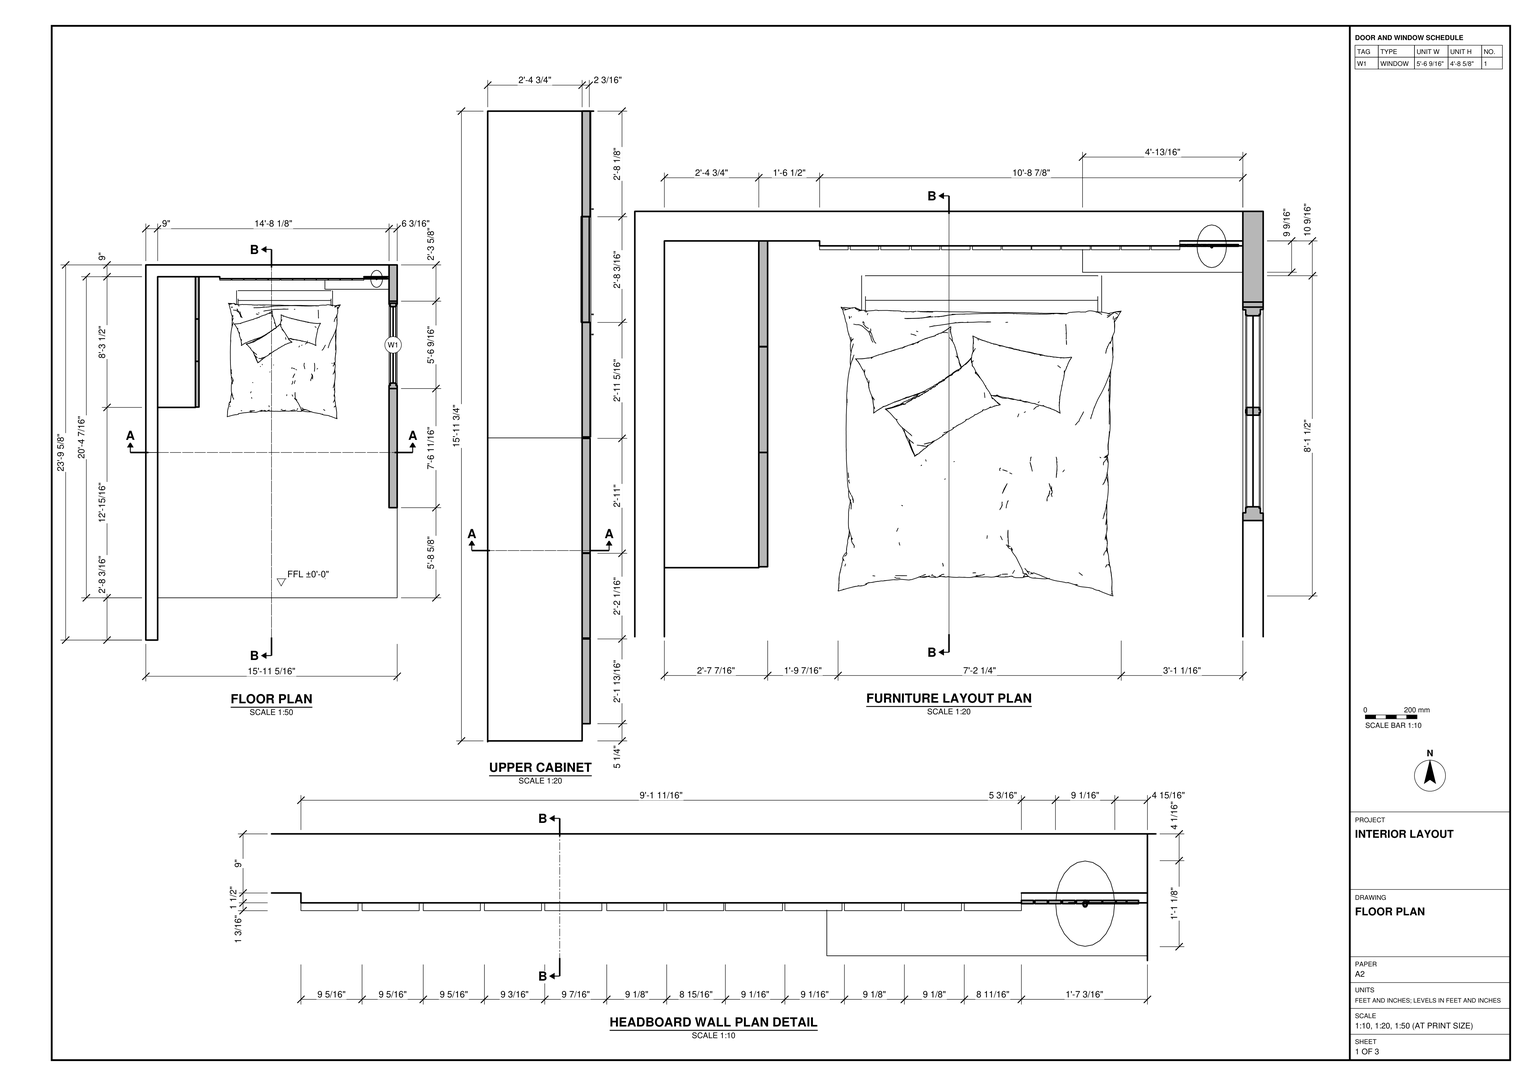
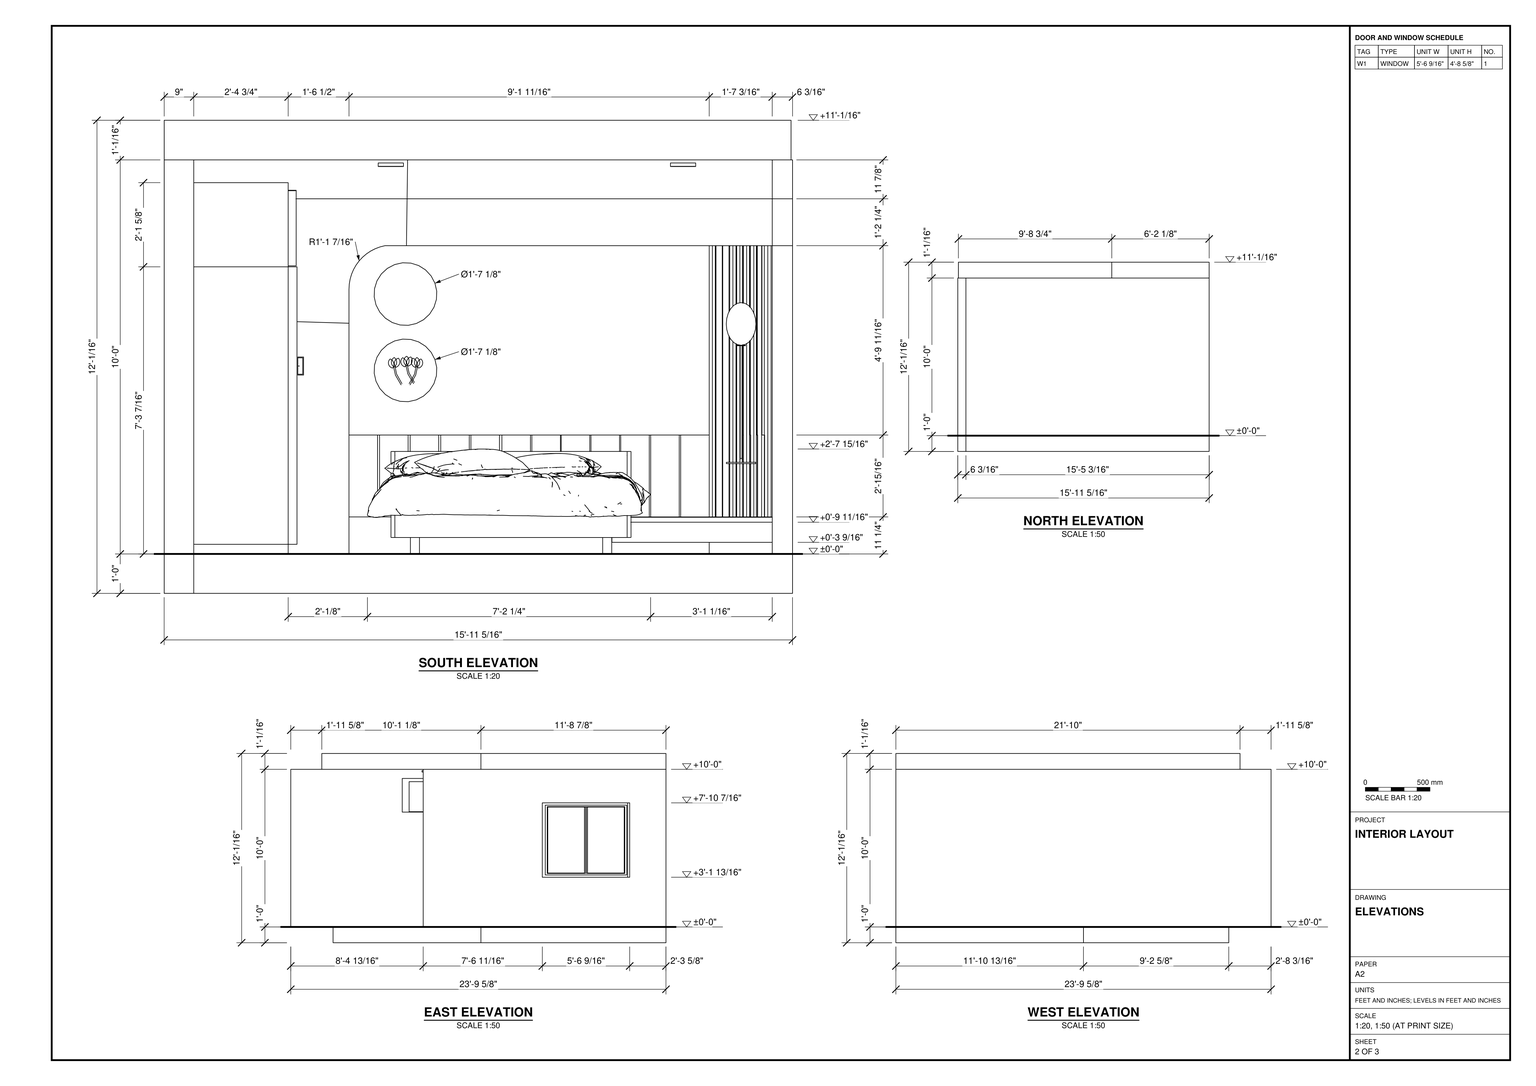
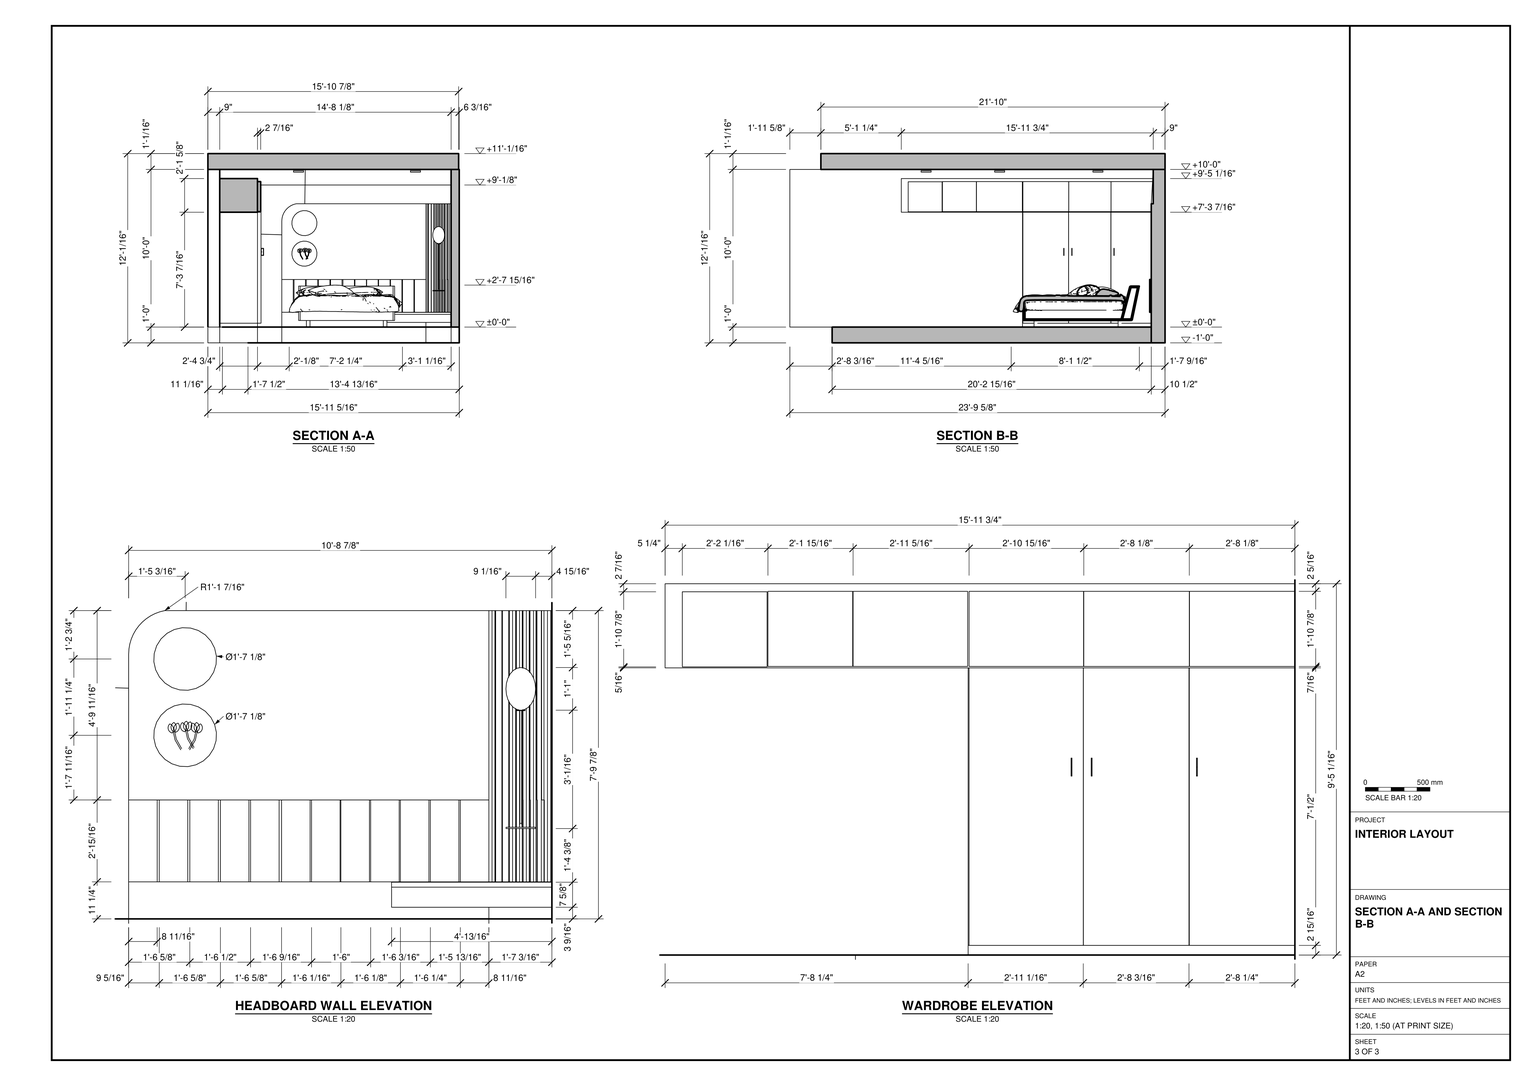
Build the bedroom interior in SketchUp using task_files/diagram_01.pdf. Work in feet and inches. The overall model is 15'-11 5/16" wide, 23'-9 5/8" long and 12'-1/16" high, with the finished floor at ±0'-0". Follow the floor plan for the wall thicknesses and unequal side-wall lengths. Leave the south end open as drawn. Use the sections to set out the floor slab and flat roof slab, noting that their ends do not align. Fit the framed window assembly into the east wall beside the bed.

Place the platform bed with its head toward the north wall, leaving the clearances shown between the bed, wardrobe and window wall. Along the west wall, model the tall wardrobe doors and handles beneath the row of upper cupboards. Continue the upper cupboards beyond the tall doors toward the open end. Behind the bed, model the broad panel with its rounded upper left corner, the divided panels below it, the narrow slatted section on the right and the low projecting shelf. Decor and loose items may be any suitable library components placed as shown.

Keep each shell element and each furniture or joinery piece in a separate group or component, and use components for repeated parts. Save one SketchUp model as output_files/bedroom_with_a_fitted_wardrobe_and_headboard_wall.skp.

# SketchUp Ruby script. Lengths in inches.
U = 1.inch
M = Sketchup.active_model
def pt(a) = Geom::Point3d.new(a.map { |v| v * U })
def face(e, loops, mat)
  f = e.add_face(loops[0].map { |a| pt(a) })
  loops[1..].each { |l| e.add_face(l.map { |a| pt(a) }).erase! }
  f.material = f.back_material = mat if mat
  f
end
# faces: each face lists its corners as indices into pts; further lists are holes
def faces(e, pts, list, mat = nil) = list.each { |f| face(e, (f[0].is_a?(Array) ? f : [f]).map { |l| l.map { |i| pts[i] } }, mat) }
# xy, xz, yz: faces in a plane at the given z, y or x. An outline is a flat list of corners, or four numbers for a rectangle; further outlines are holes
def ring(l) = l.size == 4 ? [[l[0], l[1]], [l[2], l[1]], [l[2], l[3]], [l[0], l[3]]] : l.each_slice(2).to_a
def flat(e, list, mat, &to3) = list.each { |f| face(e, (f[0].is_a?(Array) ? f : [f]).map { |l| ring(l).map { |u, v| to3.(u, v) } }, mat) }
def xy(e, z, list, mat = nil) = flat(e, list, mat) { |x, y| [x, y, z] }
def xz(e, y, list, mat = nil) = flat(e, list, mat) { |x, z| [x, y, z] }
def yz(e, x, list, mat = nil) = flat(e, list, mat) { |y, z| [x, y, z] }
def lines(e, pts, list) = list.each { |a, b| e.add_line(pt(pts[a]), pt(pts[b])) }
# prism: a flat outline (further loops are holes) pulled along v
def prism(e, loops, v, mat = nil)
  f = face(e, loops, mat); d = Geom::Vector3d.new(v.map { |x| x * U })
  f.pushpull(f.normal.samedirection?(d) ? d.length : -d.length)
end
def box(e, o, s, mat = nil) = prism(e, [[o, [o[0] + s[0], o[1], o[2]], [o[0] + s[0], o[1] + s[1], o[2]], [o[0], o[1] + s[1], o[2]]]], [0, 0, s[2]], mat)
def at(x, y, z, deg = 0) = Geom::Transformation.translation(pt([x, y, z])) * Geom::Transformation.rotation(ORIGIN, Z_AXIS, deg.degrees)
def axes(o, x, y, z) = Geom::Transformation.new([*x, 0, *y, 0, *z, 0, *pt(o).to_a, 1])
def part(name) = M.definitions.add(name)
# library, detail: a bought-in or finely detailed component or shape, given as its bounding box
def library(name, o, s) = part(name).tap { |d| box(d.entities, o, s) }
def detail(e, o, s) = box(e.add_group.entities, o, s)
def put(e, d, t, mat = nil) = e.add_instance(d, t).tap { |i| i.material = mat if mat }
def group(e, t, mat = nil) = e.add_group.tap { |g| g.transformation = t; g.material = mat if mat }.entities
root = M.entities
M.materials.add("[Carrera Marble]").color = [207, 207, 207]
M.materials.add("[Color A02]").color = [255, 153, 153]
M.materials.add("[Color M03]").color = [170, 170, 170]
M.materials.add("[CoolGray8]").color = [76, 80, 93]
M.materials.add("[Translucent Glass Gray]").color = [128, 128, 128]
M.materials["[Translucent Glass Gray]"].alpha = 0.5
M.materials.add("[Wood Cherry Original]").color = [152, 86, 42]
M.materials.add("[Wood Floor]").color = [155, 105, 61]
c1 = library("BED+04",[-44.14,-47.125,0],[86.23,97.52,31.95])
c2 = part("window full")
xy(c2.entities,0,[[0,0,14.17,66.54]])
xy(c2.entities,2.26,[[12.2,2.26,14.17,64.28]],"[Wood Floor]")
xy(c2.entities,2.36,[[0,2.36,1.97,64.17]],"[Wood Floor]")
xy(c2.entities,3.74,[[11.42,3.74,12.2,32.875],[11.42,33.66,12.2,62.79]],"[Wood Floor]")
xy(c2.entities,3.9375,[[1.97,3.9375,2.76,32.77],[1.97,33.76,2.76,62.6]],"[Wood Floor]")
xy(c2.entities,4.18,[[2.76,4.18,7.09,32.09],[7.09,4.18,11.42,32.09],[2.76,34.45,7.09,62.35],[7.09,34.45,11.42,62.35]],"[Wood Floor]")
xy(c2.entities,69.83,[[2.76,4.18,7.09,32.09],[7.09,32.09,11.42,34.45],[2.76,34.45,7.09,62.35]])
xy(c2.entities,69.83,[[7.09,4.18,11.42,32.09],[7.09,34.45,11.42,62.35]],"[Wood Floor]")
xy(c2.entities,70.08,[[1.97,3.9375,2.76,32.77],[1.97,33.76,2.76,62.6]])
xy(c2.entities,70.27,[[11.42,32.875,12.2,33.66]])
xy(c2.entities,70.27,[[11.42,3.74,12.2,32.875],[11.42,33.66,12.2,62.79]],"[Wood Floor]")
xy(c2.entities,71.65,[[0,2.36,1.97,64.17]])
xy(c2.entities,71.76,[[12.2,2.26,14.17,64.28]],"[Wood Floor]")
xy(c2.entities,74.02,[[0,0,14.17,66.54]],"[Wood Floor]")
xz(c2.entities,0,[[0,0,14.17,74.02]],"[Wood Floor]")
xz(c2.entities,2.26,[[12.2,2.26,14.17,71.76]],"[Wood Floor]")
xz(c2.entities,2.36,[[0,2.36,1.97,71.65]],"[Wood Floor]")
xz(c2.entities,3.74,[[11.42,3.74,12.2,70.27]],"[Wood Floor]")
xz(c2.entities,3.9375,[[1.97,3.9375,2.76,70.08]],"[Wood Floor]")
xz(c2.entities,4.18,[[2.76,4.18,7.09,69.83],[7.09,4.18,11.42,69.83]],"[Wood Floor]")
xz(c2.entities,32.09,[[2.76,4.18,11.42,69.83]],"[Wood Floor]")
xz(c2.entities,32.77,[[1.97,3.9375,2.76,70.08]],"[Wood Floor]")
xz(c2.entities,32.875,[[11.42,3.74,12.2,70.27]],"[Wood Floor]")
xz(c2.entities,33.66,[[11.42,3.74,12.2,47.88],[11.42,47.88,12.2,70.27]],"[Wood Floor]")
xz(c2.entities,33.76,[[1.97,3.9375,2.76,70.08]],"[Wood Floor]")
xz(c2.entities,34.45,[[2.76,4.18,11.42,69.83]],"[Wood Floor]")
xz(c2.entities,62.35,[[2.76,4.18,7.09,69.83],[7.09,4.18,11.42,69.83]],"[Wood Floor]")
xz(c2.entities,62.6,[[1.97,3.9375,2.76,70.08]],"[Wood Floor]")
xz(c2.entities,62.79,[[11.42,3.74,12.2,70.27]],"[Wood Floor]")
xz(c2.entities,64.17,[[0,2.36,1.97,71.65]],"[Wood Floor]")
xz(c2.entities,64.28,[[12.2,2.26,14.17,71.76]],"[Wood Floor]")
xz(c2.entities,66.54,[[0,0,14.17,74.02]],"[Wood Floor]")
yz(c2.entities,0,[[[0,0,66.54,74.02],[2.36,2.36,64.17,71.65]]],"[Wood Floor]")
yz(c2.entities,1.97,[[[2.36,2.36,64.17,71.65],[33.76,3.9375,62.6,70.08],[3.9375,3.9375,32.77,70.08]]],"[Wood Floor]")
yz(c2.entities,2.76,[[32.77,3.9375,33.76,4.18],[32.77,4.18,33.76,69.83],[32.77,69.83,33.76,70.08]])
yz(c2.entities,2.76,[[[3.9375,3.9375,32.77,70.08],[4.18,4.18,32.09,69.83]],[[33.76,3.9375,62.6,70.08],[34.45,4.18,62.35,69.83]]],"[Wood Floor]")
yz(c2.entities,7.09,[[4.18,4.18,62.35,69.83]],"[Translucent Glass Gray]")
yz(c2.entities,11.42,[[32.875,69.83,33.66,70.27]])
yz(c2.entities,11.42,[[[3.74,3.74,32.875,70.27],[4.18,4.18,32.09,69.83]],[[33.66,3.74,62.79,70.27],[34.45,4.18,62.35,69.83]]],"[Wood Floor]")
yz(c2.entities,12.2,[[[2.26,2.26,64.28,71.76],[3.74,3.74,32.875,70.27],[33.66,3.74,62.79,70.27]]],"[Wood Floor]")
yz(c2.entities,14.17,[[[0,0,66.54,74.02],[2.26,2.26,64.28,71.76]]],"[Wood Floor]")
p = [[11.42,32.875,70.27],[11.42,32.875,70.28]]
lines(c2.entities,p,[[0,1]])
c3 = library("stand lighting1",[-0.05,-6.55,3.35],[13.1,13.1,49.02])
c4 = part("Handle")
prism(c4.entities,[[[0,0,5.25],[0,0,5.5],[0,1.75,5.5],[0,1.75,0],[0,0,0],[0,0,0.25],[0,1.5,0.25],[0,1.5,5.25]]],[0.25,0,0],"[CoolGray8]")
p = [[0.25,0,0.25],[0.25,0,2.75],[0,0,0.25],[0,0,2.75],[0.25,0,5.25],[0,0,5.25],
  [0.125,0,2.75],[0.125,0.5,2.75]]
lines(c4.entities,p,[[0,1],[2,3],[1,4],[3,5],[1,6],[6,3],[6,7]])
c5 = part("グループ\#88")
xy(c5.entities,0,[[5.91,0,4.38,0.2,2.95,0.79,1.73,1.73,0.79,2.95,0.2,4.38,0,5.91,0.2,7.43,0.79,8.86,1.73,10.08,2.95,11.02,4.38,11.61,5.91,11.8125,7.43,11.61,8.86,11.02,10.08,10.08,11.02,8.86,11.61,7.43,11.8125,5.91,11.61,4.38,11.02,2.95,10.08,1.73,8.86,0.79,7.43,0.2]])
xy(c5.entities,1.57,[[5.91,0.41,7.33,0.6,8.65,1.15,9.79,2.02,10.67,3.16,11.21,4.48,11.4,5.91,11.21,7.33,10.67,8.65,9.79,9.79,8.65,10.67,7.33,11.21,5.91,11.4,4.48,11.21,3.16,10.67,2.02,9.79,1.15,8.65,0.6,7.33,0.41,5.91,0.6,4.48,1.15,3.16,2.02,2.02,3.16,1.15,4.48,0.6]])
xy(c5.entities,1.69,[[[5.91,0,7.43,0.2,8.86,0.79,10.08,1.73,11.02,2.95,11.61,4.38,11.8125,5.91,11.61,7.43,11.02,8.86,10.08,10.08,8.86,11.02,7.43,11.61,5.91,11.8125,4.38,11.61,2.95,11.02,1.73,10.08,0.79,8.86,0.2,7.43,0,5.91,0.2,4.38,0.79,2.95,1.73,1.73,2.95,0.79,4.38,0.2],[5.91,0.41,4.48,0.6,3.16,1.15,2.02,2.02,1.15,3.16,0.6,4.48,0.41,5.91,0.6,7.33,1.15,8.65,2.02,9.79,3.16,10.67,4.48,11.21,5.91,11.4,7.33,11.21,8.65,10.67,9.79,9.79,10.67,8.65,11.21,7.33,11.4,5.91,11.21,4.48,10.67,3.16,9.79,2.02,8.65,1.15,7.33,0.6]]])
p = [[4.38,0.2,0],[5.91,0,0],[5.91,0,1.69],[4.38,0.2,1.69],[7.43,0.2,0],[7.43,0.2,1.69],
  [2.95,0.79,0],[2.95,0.79,1.69],[8.86,0.79,0],[8.86,0.79,1.69],[1.73,1.73,0],[1.73,1.73,1.69],
  [10.08,1.73,0],[10.08,1.73,1.69],[0.79,2.95,0],[0.79,2.95,1.69],[11.02,2.95,0],[11.02,2.95,1.69],
  [0.2,4.38,0],[0.2,4.38,1.69],[11.61,4.38,0],[11.61,4.38,1.69],[0,5.91,0],[0,5.91,1.69],
  [11.8125,5.91,0],[11.8125,5.91,1.69],[0.2,7.43,0],[0.2,7.43,1.69],[11.61,7.43,0],[11.61,7.43,1.69],
  [0.79,8.86,0],[0.79,8.86,1.69],[11.02,8.86,0],[11.02,8.86,1.69],[1.73,10.08,0],[1.73,10.08,1.69],
  [10.08,10.08,0],[10.08,10.08,1.69],[2.95,11.02,0],[2.95,11.02,1.69],[8.86,11.02,0],[8.86,11.02,1.69],
  [4.38,11.61,0],[4.38,11.61,1.69],[7.43,11.61,0],[7.43,11.61,1.69],[5.91,11.8125,0],[5.91,11.8125,1.69],
  [4.48,0.6,1.69],[5.91,0.41,1.69],[5.91,0.41,1.57],[4.48,0.6,1.57],[7.33,0.6,1.69],[7.33,0.6,1.57],
  [3.16,1.15,1.69],[3.16,1.15,1.57],[8.65,1.15,1.69],[8.65,1.15,1.57],[2.02,2.02,1.69],[2.02,2.02,1.57],
  [9.79,2.02,1.69],[9.79,2.02,1.57],[1.15,3.16,1.69],[1.15,3.16,1.57],[10.67,3.16,1.69],[10.67,3.16,1.57],
  [0.6,4.48,1.69],[0.6,4.48,1.57],[11.21,4.48,1.69],[11.21,4.48,1.57],[0.41,5.91,1.69],[0.41,5.91,1.57],
  [11.4,5.91,1.69],[11.4,5.91,1.57],[0.6,7.33,1.69],[0.6,7.33,1.57],[11.21,7.33,1.69],[11.21,7.33,1.57],
  [1.15,8.65,1.69],[1.15,8.65,1.57],[10.67,8.65,1.69],[10.67,8.65,1.57],[2.02,9.79,1.69],[2.02,9.79,1.57],
  [9.79,9.79,1.69],[9.79,9.79,1.57],[3.16,10.67,1.69],[3.16,10.67,1.57],[8.65,10.67,1.69],[8.65,10.67,1.57],
  [4.48,11.21,1.69],[4.48,11.21,1.57],[7.33,11.21,1.69],[7.33,11.21,1.57],[5.91,11.4,1.69],[5.91,11.4,1.57]]
faces(c5.entities,p,[[0,1,2,3],[1,4,5,2],[6,0,3,7],[4,8,9,5],[10,6,7,11],[8,12,13,9],[14,10,11,15],[12,16,17,13],
  [18,14,15,19],[16,20,21,17],[22,18,19,23],[20,24,25,21],[26,22,23,27],[24,28,29,25],[30,26,27,31],[28,32,33,29],
  [34,30,31,35],[32,36,37,33],[38,34,35,39],[36,40,41,37],[42,38,39,43],[40,44,45,41],[46,42,43,47],[44,46,47,45],
  [48,49,50,51],[49,52,53,50],[54,48,51,55],[52,56,57,53],[58,54,55,59],[56,60,61,57],[62,58,59,63],[60,64,65,61],
  [66,62,63,67],[64,68,69,65],[70,66,67,71],[68,72,73,69],[74,70,71,75],[72,76,77,73],[78,74,75,79],[76,80,81,77],
  [82,78,79,83],[80,84,85,81],[86,82,83,87],[84,88,89,85],[90,86,87,91],[88,92,93,89],[94,90,91,95],[92,94,95,93]])
c6 = part("CL OL251733")
put(c6.entities,c5,axes([4.91,11.8125,72.56],[1,0,0],[0,-1,0],[0,0,-1]))
c7 = part("Group\#2")
box(c7.entities,[0,-1.1875,0],[8.69,1.1875,24.94])
c8 = part("Group\#17")
prism(c8.entities,[[[0,32.15,67.88],[0,32.15,0],[0,0,0],[0,0,84.5],[0,32.15,84.5]]],[2.6875,0,0])
c9 = part("Group\#21")
box(c9.entities,[0,0,0],[2.4375,34.875,22.875])
c10 = part("Group\#16")
box(c10.entities,[0,0,0],[2.4375,32.1875,22.875])
c11 = part("Group\#20")
box(c11.entities,[0,9.06,0],[2.4375,25.82,22.875])
c12 = part("Group\#22")
xy(c12.entities,0,[[0.875,0,1.09,0.18,1.27,0.39,1.42,0.63,1.53,0.89,1.6,1.16,1.62,1.4375,1.6,1.72,1.53,1.99,1.42,2.25,1.27,2.48,1.09,2.7,0.875,2.875,0.625,2.72,0.41,2.52,0.24,2.28,0.11,2.01,0.03,1.73,0,1.4375,0.03,1.14,0.11,0.86,0.24,0.6,0.41,0.36,0.625,0.16]])
xy(root,-12,[[9,32.1875,9,276.625,56.27,276.625,56.27,275.125,185.15,275.125,185.15,144.75,191.34,144.75,191.34,32.1875],[0,142.8125,0,285.625,185.15,285.625,185.15,276.625,165.96,276.625,165.96,275.125,56.27,275.125,56.27,276.625,9,276.625,9,142.8125],[185.15,144.75,191.34,285.625]])
xy(root,0,[[0,0,9,142.8125],[9,32.1875,191.34,32.1875,191.34,100.8125,185.15,100.8125,185.15,275.125,56.27,275.125,56.27,276.625,9,276.625],[185.15,100.8125,191.34,144.75],[165.96,275.125,185.15,276.625]])
xy(root,3.54,[[136.34,267.0625,165.96,275.125],[165.96,267.0625,185.15,275.125]])
xy(root,9.66,[[136.34,267.0625,185.15,275.125]])
xy(root,11.16,[[136.34,267.0625,185.15,275.125]],"[Wood Cherry Original]")
xy(root,37.84,[[185.15,191.47,191.34,256.47]])
xy(root,93.875,[[67.22,275.125,165.96,276.625],[165.96,275.125,185.15,276.625]])
xy(root,94.47,[[185.15,191.47,191.34,256.47]])
xy(root,120,[[0,0,9,23.625],[0,23.625,9,276.625],[9,23.625,9,276.625,185.15,276.625,185.15,100.8125,190.875,100.8125,190.875,23.625],[185.15,100.8125,190.875,285.625],[190.875,100.8125,191.34,285.625],
  [0,276.625,74.125,285.625],[74.125,276.625,185.15,285.625]])
xy(root,132.0625,[[0,23.625,190.875,285.625]])
xz(root,0,[[0,0,9,120]])
xz(root,23.625,[[0,120,190.875,132.0625]])
xz(root,32.1875,[[9,-12,191.34,0]])
xz(root,100.8125,[[185.15,0,191.34,93.875],[185.15,93.875,191.34,108.15],[185.15,108.15,191.34,120]])
xz(root,142.8125,[[0,-12,9,0]])
xz(root,144.75,[[185.15,-12,191.34,0]])
xz(root,191.47,[[185.15,37.84,191.34,94.47]])
xz(root,256.47,[[185.15,37.84,191.34,94.47]])
xz(root,267.0625,[[136.34,3.54,185.15,9.66]])
xz(root,267.0625,[[136.34,9.66,185.15,11.16]],"[Wood Cherry Original]")
xz(root,275.125,[[56.27,-12,165.96,0],[165.96,-12,185.15,0],[136.34,9.66,185.15,11.16],[64.96,11.27,165.96,36.22],[74.32,69.625,76.76,70.17,78.97,71.33,80.81,73.02,82.14,75.13,82.89,77.51,82.99,80.01,82.44,82.44,81.28,84.65,79.59,86.49,77.48,87.83,75.1,88.57,72.61,88.67,70.17,88.125,67.96,86.97,66.12,85.28,64.79,83.17,64.04,80.78,63.94,78.29,64.49,75.85,65.65,73.64,67.34,71.81,69.45,70.47,71.83,69.73]])
xz(root,275.125,[[[56.27,36.22,165.96,36.22,165.96,93.875,67.22,93.875,65.72,93.5,64.27,92.96,62.89,92.25,61.6,91.39,60.42,90.38,59.36,89.25,58.44,88,57.68,86.65,57.07,85.23,56.625,83.74,56.36,82.22,56.27,80.67],[74.32,69.625,71.83,69.73,69.45,70.47,67.34,71.81,65.65,73.64,64.49,75.85,63.94,78.29,64.04,80.78,64.79,83.17,66.12,85.28,67.96,86.97,70.17,88.125,72.61,88.67,75.1,88.57,77.48,87.83,79.59,86.49,81.28,84.65,82.44,82.44,82.99,80.01,82.89,77.51,82.14,75.13,80.81,73.02,78.97,71.33,76.76,70.17],[75.49,52.59,75.24,53.03,75.49,53.47,75.74,53.02]],[75.49,52.59,75.74,53.02,75.49,53.47,75.24,53.03]],"[Color A02]")
xz(root,275.125,[[56.27,0,165.96,0,165.96,3.54,136.34,3.54,136.34,11.16,185.15,11.16,185.15,11.27,56.27,11.27],[165.96,0,185.15,3.54],[173.17,11.27,174.23,93.875],[175.3,11.27,176.36,93.875],[176.36,11.27,177.36,93.875],
  [177.36,11.27,178.48,93.875],[178.48,11.27,179.55,93.875],[179.55,11.27,180.61,93.875],[180.61,11.27,182.73,93.875],[182.73,11.27,183.8,93.875],
  [183.8,11.27,184.8,93.875],[184.8,11.27,185.15,93.875]],"[Wood Cherry Original]")
xz(root,276.625,[[9,-12,37.75,0],[37.75,-12,56.27,0],[165.96,-12,185.15,0]])
xz(root,276.625,[[9,0,56.27,0,56.27,80.67,56.36,82.22,56.625,83.74,57.07,85.23,57.68,86.65,58.44,88,59.36,89.25,60.42,90.38,61.6,91.39,62.89,92.25,64.27,92.96,65.72,93.5,67.22,93.875,185.15,93.875,185.15,108.15,9,108.15],[9,108.15,185.15,120]],"[Carrera Marble]")
xz(root,276.625,[[165.96,0,185.15,93.875]],"[Wood Cherry Original]")
xz(root,285.625,[[0,-12,185.15,120],[185.15,-12,191.34,120],[0,120,74.125,132.0625],[74.125,120,190.875,132.0625]])
yz(root,0,[[142.8125,-12,142.8125,0,0,0,0,120,285.625,120,285.625,-12],[23.625,120,285.625,132.0625]])
yz(root,9,[[32.1875,-12,142.8125,0],[142.8125,-12,276.625,0],[0,0,276.625,120]])
yz(root,56.27,[[275.125,-12,276.625,0],[275.125,0,276.625,80.67]])
yz(root,136.34,[[267.0625,3.54,275.125,9.66],[267.0625,9.66,275.125,11.16]])
yz(root,165.96,[[275.125,-12,276.625,0]])
yz(root,185.15,[[144.75,-12,275.125,0],[275.125,-12,276.625,0],[276.625,-12,285.625,120],[[100.8125,0,100.8125,120,276.625,120,276.625,93.875,275.125,93.875,275.125,11.16,267.0625,11.16,267.0625,3.54,275.125,3.54,275.125,0],[191.47,37.84,256.47,94.47]],[275.125,0,275.125,3.54,267.0625,3.54,267.0625,9.66,275.125,9.66,275.125,93.875,276.625,93.875,276.625,0],
  [267.0625,9.66,275.125,11.16]])
yz(root,185.15,[[267.0625,9.66,275.125,11.16]],"[Wood Cherry Original]")
yz(root,190.875,[[23.625,120,144.75,132.0625],[144.75,120,285.625,132.0625]])
yz(root,191.34,[[32.1875,-12,144.75,0],[[144.75,-12,285.625,-12,285.625,120,100.8125,120,100.8125,0,144.75,0],[191.47,37.84,256.47,94.47]]])
p = [[56.36,276.625,82.22],[56.27,276.625,80.67],[56.27,275.125,80.67],[56.36,275.125,82.22],[56.625,276.625,83.74],[56.625,275.125,83.74],
  [57.07,276.625,85.23],[57.07,275.125,85.23],[57.68,276.625,86.65],[57.68,275.125,86.65],[58.44,276.625,88],[58.44,275.125,88],
  [59.36,276.625,89.25],[59.36,275.125,89.25],[60.42,276.625,90.38],[60.42,275.125,90.38],[61.6,276.625,91.39],[61.6,275.125,91.39],
  [62.89,276.625,92.25],[62.89,275.125,92.25],[64.27,276.625,92.96],[64.27,275.125,92.96],[65.72,276.625,93.5],[65.72,275.125,93.5],
  [67.22,276.625,93.875],[67.22,275.125,93.875],[166.92,275.125,93.875],[166.92,275.125,11.27],[167.92,275.125,93.875],[167.92,275.125,11.27],
  [73.76,275.125,93.875],[74.125,276.625,120],[37.75,276.625,70.82],[56.27,276.625,70.25],[69.82,275.125,57.09],[70.41,275.125,54.46],
  [72.13,275.125,51.49],[70.26,275.125,57.13],[70.78,275.125,54.75],[72.4,275.125,51.86],[77.16,275.125,57.09],[76.57,275.125,54.46],
  [76.72,275.125,57.13],[76.2,275.125,54.75],[75.49,275.125,53.47],[75.74,275.125,53.02],[74.19,275.125,54.85],[75.24,275.125,53.03],
  [73.6,275.125,57.47],[74.56,275.125,55.13],[74.04,275.125,57.51],[74.59,275.125,51.86],[75.49,275.125,52.59],[74.85,275.125,51.49],
  [75.91,275.125,51.87],[76.18,275.125,52.24]]
faces(root,p,[[0,1,2,3],[4,0,3,5],[6,4,5,7],[8,6,7,9],[10,8,9,11],[12,10,11,13],[14,12,13,15],[16,14,15,17],
  [18,16,17,19],[20,18,19,21],[22,20,21,23],[24,22,23,25]])
lines(root,p,[[26,27],[28,29],[30,31],[32,33],[34,35],[35,36],[37,38],[38,39],[40,41],[42,43],[43,44],[41,45],
  [46,47],[48,46],[49,44],[50,49],[47,51],[52,53],[52,54],[45,55]])
put(root,c1,at(106.01,215.63,0))
put(root,c2,axes([185.15,191.47,37.84],[0.43656,0,0],[0,1,0],[0,0,0.76504]))
put(root,c3,axes([171.18,275,24.16],[0.68979,0,0],[0,1,0],[0,0,1]))
put(root,c4,at(40.69,214.87,54.48,-91.014))
put(root,c4,at(40.69,208.75,54.48,-91.014))
put(root,c4,at(40.69,246.93,54.48,-91.014))
put(root,c6,axes([61.97,230.7,71.9],[0.65,0,0],[0,0.65,0],[0,0,0.65]))
put(root,c6,axes([150.97,230.7,71.9],[0.65,0,0],[0,0.65,0],[0,0,0.65]))
put(root,c6,axes([61.97,155.88,71.9],[0.65,0,0],[0,0.65,0],[0,0,0.65]))
put(root,c6,axes([150.97,155.88,71.9],[0.65,0,0],[0,0.65,0],[0,0,0.65]))
put(root,c6,axes([150.97,99.88,71.9],[0.65,0,0],[0,0.65,0],[0,0,0.65]))
put(root,c6,axes([61.97,99.88,71.9],[0.65,0,0],[0,0.65,0],[0,0,0.65]))
put(root,c7,at(56.27,275.125,11.27),"[Color M03]")
put(root,c7,at(65.58,275.125,11.27),"[Color M03]")
put(root,c7,at(74.89,275.125,11.27),"[Color M03]")
put(root,c7,at(84.21,275.125,11.27),"[Color M03]")
put(root,c7,at(93.39,275.125,11.27),"[Color M03]")
put(root,c7,at(102.83,275.125,11.27),"[Color M03]")
put(root,c7,at(111.96,275.125,11.27),"[Color M03]")
put(root,c7,at(120.89,275.125,11.27),"[Color M03]")
put(root,c7,at(129.96,275.125,11.27),"[Color M03]")
put(root,c7,at(139.02,275.125,11.27),"[Color M03]")
put(root,c7,at(148.14,275.125,11.27),"[Color M03]")
put(root,c7,at(157.27,275.125,11.27),"[Color M03]")
g1 = group(root,at(165.96,275.125,11.27),"[Wood Cherry Original]")
prism(g1,[[[0,-0.125,0],[1.84,-0.125,0],[1.84,-0.125,82.6],[0,-0.125,82.6],[0,-0.125,24.94]]],[0,0.5,0])
g2 = group(root,at(168.02,275.125,11.27),"[Wood Cherry Original]")
prism(g2,[[[0,-0.125,0],[1.9,-0.125,0],[1.9,-0.125,82.6],[0,-0.125,82.6],[0,-0.125,24.94]]],[0,0.5,0])
g3 = group(root,at(170.09,275.125,11.27),"[Wood Cherry Original]")
prism(g3,[[[0,-0.125,0],[1.9,-0.125,0],[1.9,-0.125,82.6],[0,-0.125,82.6],[0,-0.125,24.94]]],[0,0.5,0])
g4 = group(root,at(172.21,275.125,11.27),"[Wood Cherry Original]")
prism(g4,[[[0,-0.125,0],[1.9,-0.125,0],[1.9,-0.125,82.6],[0,-0.125,82.6],[0,-0.125,24.94]]],[0,0.5,0])
g5 = group(root,at(174.34,275.125,11.27),"[Wood Cherry Original]")
prism(g5,[[[0,-0.125,0],[1.77,-0.125,0],[1.77,-0.125,82.6],[0,-0.125,82.6],[0,-0.125,24.94]]],[0,0.5,0])
g6 = group(root,at(176.4,275.125,11.27),"[Wood Cherry Original]")
prism(g6,[[[0,-0.125,0],[1.84,-0.125,0],[1.84,-0.125,82.6],[-0.1875,-0.125,82.6],[-0.1875,-0.125,24.94],[0,-0.125,24.94]]],[0,0.5,0])
g7 = group(root,at(178.59,275.125,11.27),"[Wood Cherry Original]")
prism(g7,[[[0,-0.125,0],[1.71,-0.125,0],[1.71,-0.125,82.6],[-0.25,-0.125,82.6],[-0.25,-0.125,24.94],[0,-0.125,24.94]]],[0,0.5,0])
g8 = group(root,at(180.71,275.125,11.27),"[Wood Cherry Original]")
prism(g8,[[[0,-0.125,0],[1.21,-0.125,0],[1.21,-0.125,82.6],[-0.3125,-0.125,82.6],[-0.3125,-0.125,24.94],[0,-0.125,24.94]]],[0,0.5,0])
g9 = group(root,at(182.84,275.125,11.27),"[Wood Cherry Original]")
prism(g9,[[[0,-0.125,0],[0.96,-0.125,0],[0.96,-0.125,82.6],[-0.8125,-0.125,82.6],[-0.8125,-0.125,24.94],[0,-0.125,24.94]]],[0,0.5,0])
g10 = group(root,at(9,132.625,0),"[Wood Cherry Original]")
xy(g10,0,[[0,44.5,28.75,144]])
xy(g10,2.9375,[[0,44.5,28.75,144]])
xy(g10,87.4375,[[0,44.5,28.75,144]])
xz(g10,44.5,[[0,0,28.75,2.9375],[0,2.9375,28.75,87.4375]])
xz(g10,144,[[0,0,28.75,2.9375],[0,2.9375,28.75,87.4375]])
yz(g10,0,[[44.5,0,144,2.9375],[44.5,2.9375,144,87.4375]])
yz(g10,28.75,[[44.5,0,144,2.9375],[44.5,2.9375,144,87.4375]])
put(root,c8,at(37.75,244.47,2.9375))
put(root,c8,at(37.75,212.22,2.9375))
g11 = group(root,at(37.75,180.03,2.9375))
prism(g11,[[[0,32.15,67.88],[0,32.15,0],[0,-2.625,0],[0,-2.625,84.5],[0,32.15,84.5]]],[2.6875,0,0])
g12 = group(root,at(9,244.47,87.4375),"[Wood Cherry Original]")
box(g12,[0,-159.625,0],[28.75,191.78,25.625])
put(root,c9,at(37.75,177.41,87.875))
put(root,c10,at(37.5,212.35,87.875))
put(root,c10,at(37.75,244.47,87.875))
put(root,c9,at(37.75,142.1,87.875))
put(root,c11,at(37.75,107.1,87.875))
put(root,c11,at(37.75,81.03,87.74))
put(root,c12,axes([69.17,275.125,56.95],[1,0,0],[0,0,1],[0,-1,0]))
put(root,c12,axes([69.75,275.125,57.07],[0.96593,0,-0.25882],[0.25882,0,0.96593],[0,-1,0]))
put(root,c12,axes([68.69,275.125,56.38],[0.96593,0,0.25882],[-0.25882,0,0.96593],[0,-1,0]))
g13 = group(root,at(63.94,275.125,46.375))
xz(g13,0,[[10.38,0,12.82,0.55,15.03,1.71,16.87,3.4,18.2,5.51,18.95,7.89,19.05,10.38,18.5,12.82,17.34,15.03,15.65,16.87,13.54,18.2,11.16,18.95,8.66,19.05,6.23,18.5,4.02,17.34,2.18,15.65,0.85,13.54,0.1,11.16,0,8.66,0.55,6.23,1.71,4.02,3.4,2.18,5.51,0.85,7.89,0.1]])
put(root,c12,axes([78.29,275.125,56.38],[-0.96593,0,0.25882],[0.25882,0,0.96593],[0,-1,0]))
put(root,c12,axes([77.24,275.125,57.07],[-0.96593,0,-0.25882],[-0.25882,0,0.96593],[0,-1,0]))
put(root,c12,axes([77.8125,275.125,56.95],[-1,0,0],[0,0,1],[0,-1,0]))
put(root,c12,axes([72.95,275.125,57.33],[1,0,0],[0,0,1],[0,-1,0]))
put(root,c12,axes([73.53,275.125,57.45],[0.96593,0,-0.25882],[0.25882,0,0.96593],[0,-1,0]))
put(root,c12,axes([72.47,275.125,56.76],[0.96593,0,0.25882],[-0.25882,0,0.96593],[0,-1,0]))
